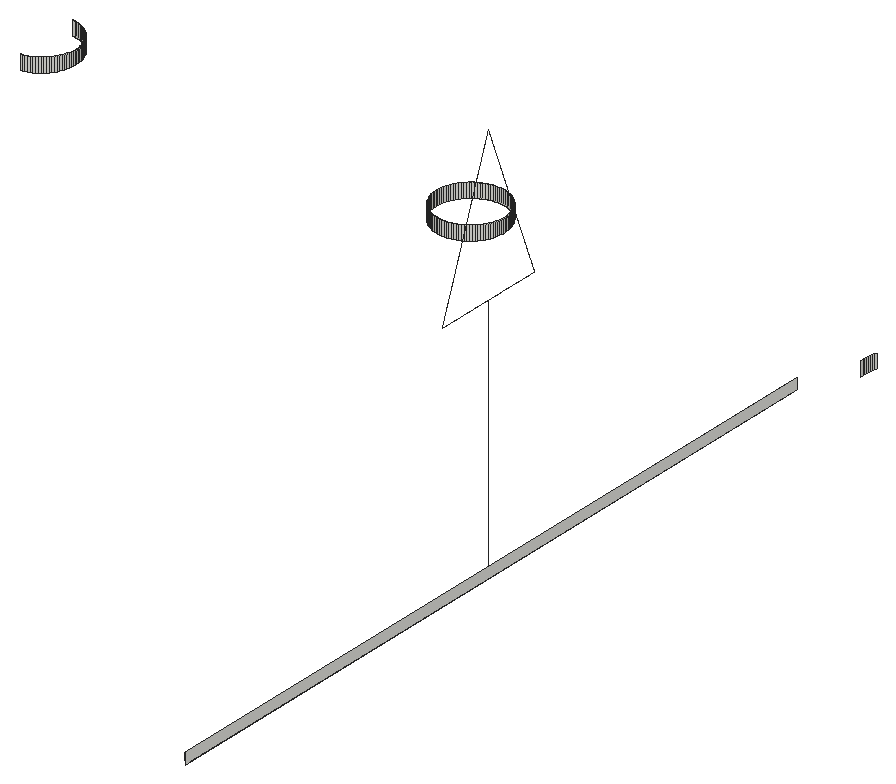
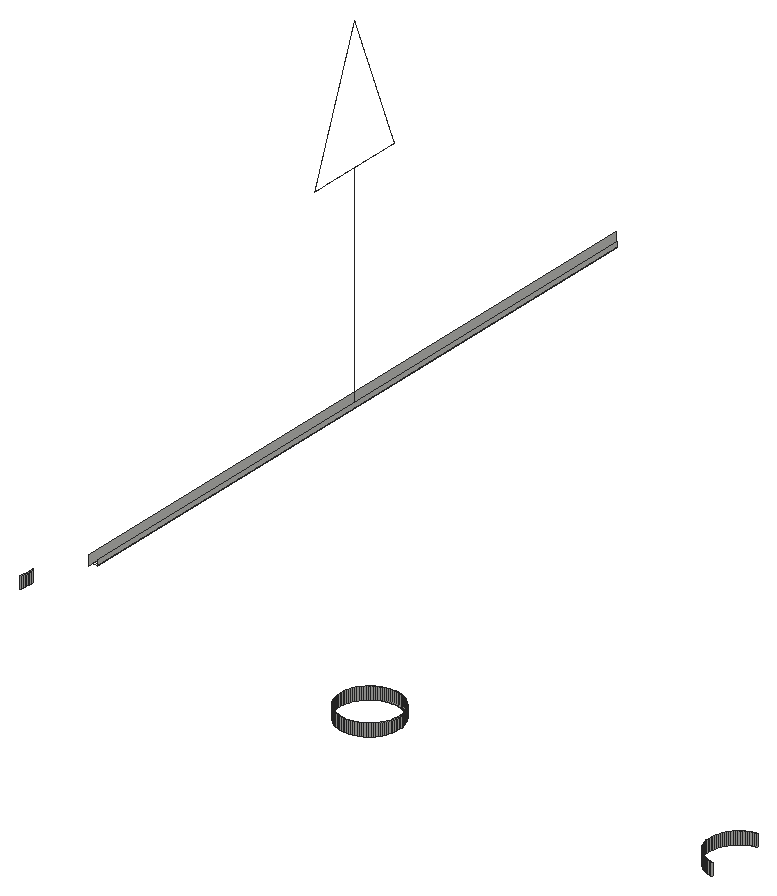
# SketchUp Ruby script. Lengths in inches.
U = 1.inch
M = Sketchup.active_model
def pt(a) = Geom::Point3d.new(a.map { |v| v * U })
def face(e, loops, mat)
  f = e.add_face(loops[0].map { |a| pt(a) })
  loops[1..].each { |l| e.add_face(l.map { |a| pt(a) }).erase! }
  f.material = f.back_material = mat if mat
  f
end
# faces: each face lists its corners as indices into pts; further lists are holes
def faces(e, pts, list, mat = nil) = list.each { |f| face(e, (f[0].is_a?(Array) ? f : [f]).map { |l| l.map { |i| pts[i] } }, mat) }
# xy, xz, yz: faces in a plane at the given z, y or x. An outline is a flat list of corners, or four numbers for a rectangle; further outlines are holes
def ring(l) = l.size == 4 ? [[l[0], l[1]], [l[2], l[1]], [l[2], l[3]], [l[0], l[3]]] : l.each_slice(2).to_a
def flat(e, list, mat, &to3) = list.each { |f| face(e, (f[0].is_a?(Array) ? f : [f]).map { |l| ring(l).map { |u, v| to3.(u, v) } }, mat) }
def xy(e, z, list, mat = nil) = flat(e, list, mat) { |x, y| [x, y, z] }
def xz(e, y, list, mat = nil) = flat(e, list, mat) { |x, z| [x, y, z] }
def yz(e, x, list, mat = nil) = flat(e, list, mat) { |y, z| [x, y, z] }
def lines(e, pts, list) = list.each { |a, b| e.add_line(pt(pts[a]), pt(pts[b])) }
# prism: a flat outline (further loops are holes) pulled along v
def prism(e, loops, v, mat = nil)
  f = face(e, loops, mat); d = Geom::Vector3d.new(v.map { |x| x * U })
  f.pushpull(f.normal.samedirection?(d) ? d.length : -d.length)
end
def box(e, o, s, mat = nil) = prism(e, [[o, [o[0] + s[0], o[1], o[2]], [o[0] + s[0], o[1] + s[1], o[2]], [o[0], o[1] + s[1], o[2]]]], [0, 0, s[2]], mat)
def at(x, y, z, deg = 0) = Geom::Transformation.translation(pt([x, y, z])) * Geom::Transformation.rotation(ORIGIN, Z_AXIS, deg.degrees)
def axes(o, x, y, z) = Geom::Transformation.new([*x, 0, *y, 0, *z, 0, *pt(o).to_a, 1])
def part(name) = M.definitions.add(name)
# library, detail: a bought-in or finely detailed component or shape, given as its bounding box
def library(name, o, s) = part(name).tap { |d| box(d.entities, o, s) }
def detail(e, o, s) = box(e.add_group.entities, o, s)
def put(e, d, t, mat = nil) = e.add_instance(d, t).tap { |i| i.material = mat if mat }
def group(e, t, mat = nil) = e.add_group.tap { |g| g.transformation = t; g.material = mat if mat }.entities
root = M.entities
c1 = part("Group84\#1")
p = [[0,0,0],[0,0,-43.36],[-21.49,0,-43.36],[139.88,-0.5,0],[-139.88,-0.5,0],[139.88,0.5,0],
  [139.88,0,0],[-139.88,0.5,0],[21.49,0,-43.36],[-139.88,0,0],[0,0,-70.19]]
lines(c1.entities,p,[[0,1],[1,2],[3,4],[5,6],[7,5],[1,8],[9,0],[0,6],[8,10],[4,9],[6,3],[2,10],
  [9,7]])
c2 = part("Rectangle Light")
put(c2.entities,c1,at(0,0,0))
xz(root,188,[[295.37,231.53,295.75,234]])
xz(root,200,[[295.37,231.53,295.75,234]])
yz(root,226.37,[[193.8125,231.53,194.1875,234]])
yz(root,289.5625,[[193.8125,231.53,194.1875,234]])
yz(root,301.56,[[193.8125,231.53,194.1875,234]])
yz(root,359.75,[[51,232,183,233]])
yz(root,360.75,[[50,232,184,234]])
yz(root,364.75,[[193.8125,231.53,194.1875,234]])
p = [[295,188.03,231.53],[294.62,188.07,231.53],[294.62,188.07,234],[295,188.03,234],[295.37,188,231.53],[295.37,188,234],
  [296.125,188.03,231.53],[295.75,188,231.53],[295.75,188,234],[296.125,188.03,234],[296.5,188.07,231.53],[296.5,188.07,234],
  [221.68,188.14,231.53],[221.31,188.07,231.53],[221.31,188.07,234],[221.68,188.14,234],[222.04,188.24,231.53],[222.04,188.24,234],
  [294.25,188.14,231.53],[293.89,188.24,231.53],[293.89,188.24,234],[294.25,188.14,234],[296.87,188.14,231.53],[296.87,188.14,234],
  [297.23,188.24,231.53],[297.23,188.24,234],[222.4,188.35,231.53],[222.4,188.35,234],[293.53,188.35,231.53],[293.53,188.35,234],
  [297.59,188.35,231.53],[297.59,188.35,234],[222.75,188.49,231.53],[222.75,188.49,234],[293.18,188.49,231.53],[293.18,188.49,234],
  [297.94,188.49,231.53],[297.94,188.49,234],[223.09,188.65,231.53],[223.09,188.65,234],[292.84,188.65,231.53],[292.84,188.65,234],
  [298.28,188.65,231.53],[298.28,188.65,234],[223.43,188.84,231.53],[223.43,188.84,234],[292.51,188.84,231.53],[292.51,188.84,234],
  [298.61,188.84,231.53],[298.61,188.84,234],[223.74,189.04,231.53],[223.74,189.04,234],[292.1875,189.04,231.53],[292.1875,189.04,234],
  [298.93,189.04,231.53],[298.93,189.04,234],[224.05,189.26,231.53],[224.05,189.26,234],[291.88,189.26,231.53],[291.88,189.26,234],
  [299.24,189.26,231.53],[299.24,189.26,234],[224.34,189.5,231.53],[224.34,189.5,234],[291.59,189.5,231.53],[291.59,189.5,234],
  [299.53,189.5,231.53],[299.53,189.5,234],[224.61,189.76,231.53],[224.61,189.76,234],[291.32,189.76,231.53],[291.32,189.76,234],
  [299.8,189.76,231.53],[299.8,189.76,234],[224.87,190.03,231.53],[224.87,190.03,234],[291.06,190.03,231.53],[291.06,190.03,234],
  [300.0625,190.03,231.53],[300.0625,190.03,234],[225.11,190.32,231.53],[225.11,190.32,234],[290.82,190.32,231.53],[290.82,190.32,234],
  [300.3,190.32,231.53],[300.3,190.32,234],[225.33,190.63,231.53],[225.33,190.63,234],[290.6,190.63,231.53],[290.6,190.63,234],
  [300.52,190.63,231.53],[300.52,190.63,234],[225.54,190.95,231.53],[225.54,190.95,234],[290.4,190.95,231.53],[290.4,190.95,234],
  [300.72,190.95,231.53],[300.72,190.95,234],[225.72,191.28,231.53],[225.72,191.28,234],[290.21,191.28,231.53],[290.21,191.28,234],
  [300.91,191.28,231.53],[300.91,191.28,234],[225.88,191.62,231.53],[225.88,191.62,234],[290.05,191.62,231.53],[290.05,191.62,234],
  [301.07,191.62,231.53],[301.07,191.62,234],[226.02,191.97,231.53],[226.02,191.97,234],[289.92,191.97,231.53],[289.92,191.97,234],
  [301.21,191.97,231.53],[301.21,191.97,234],[226.13,192.33,231.53],[226.13,192.33,234],[289.8,192.33,231.53],[289.8,192.33,234],
  [301.32,192.33,231.53],[301.32,192.33,234],[226.23,192.69,231.53],[226.23,192.69,234],[289.7,192.69,231.53],[289.7,192.69,234],
  [301.42,192.69,231.53],[301.42,192.69,234],[226.3,193.0625,231.53],[226.3,193.0625,234],[289.63,193.0625,231.53],[289.63,193.0625,234],
  [301.49,193.0625,231.53],[301.49,193.0625,234],[226.34,193.44,231.53],[226.34,193.44,234],[289.59,193.44,231.53],[289.59,193.44,234],
  [301.53,193.44,231.53],[301.53,193.44,234],[364.82,193.0625,231.53],[364.78,193.44,231.53],[364.78,193.44,234],[364.82,193.0625,234],
  [226.37,193.8125,231.53],[226.37,193.8125,234],[289.5625,193.8125,231.53],[289.5625,193.8125,234],[301.56,193.8125,231.53],[301.56,193.8125,234],
  [364.75,193.8125,231.53],[364.75,193.8125,234],[226.34,194.56,231.53],[226.37,194.1875,231.53],[226.37,194.1875,234],[226.34,194.56,234],
  [289.5625,194.1875,231.53],[289.59,194.56,231.53],[289.59,194.56,234],[289.5625,194.1875,234],[301.53,194.56,231.53],[301.56,194.1875,231.53],
  [301.56,194.1875,234],[301.53,194.56,234],[364.75,194.1875,231.53],[364.78,194.56,231.53],[364.78,194.56,234],[364.75,194.1875,234],
  [226.3,194.9375,231.53],[226.3,194.9375,234],[289.63,194.9375,231.53],[289.63,194.9375,234],[301.49,194.9375,231.53],[301.49,194.9375,234],
  [364.82,194.9375,231.53],[364.82,194.9375,234],[226.23,195.31,231.53],[226.23,195.31,234],[289.7,195.31,231.53],[289.7,195.31,234],
  [301.42,195.31,231.53],[301.42,195.31,234],[364.89,195.31,231.53],[364.89,195.31,234],[226.13,195.67,231.53],[226.13,195.67,234],
  [289.8,195.67,231.53],[289.8,195.67,234],[301.32,195.67,231.53],[301.32,195.67,234],[364.99,195.67,231.53],[364.99,195.67,234],
  [226.02,196.03,231.53],[226.02,196.03,234],[289.92,196.03,231.53],[289.92,196.03,234],[301.21,196.03,231.53],[301.21,196.03,234],
  [365.1,196.03,231.53],[365.1,196.03,234],[225.88,196.38,231.53],[225.88,196.38,234],[290.05,196.38,231.53],[290.05,196.38,234],
  [301.07,196.38,231.53],[301.07,196.38,234],[225.72,196.72,231.53],[225.72,196.72,234],[290.21,196.72,231.53],[290.21,196.72,234],
  [300.91,196.72,231.53],[300.91,196.72,234],[225.54,197.05,231.53],[225.54,197.05,234],[290.4,197.05,231.53],[290.4,197.05,234],
  [300.72,197.05,231.53],[300.72,197.05,234],[225.33,197.37,231.53],[225.33,197.37,234],[290.6,197.37,231.53],[290.6,197.37,234],
  [300.52,197.37,231.53],[300.52,197.37,234],[225.11,197.68,231.53],[225.11,197.68,234],[290.82,197.68,231.53],[290.82,197.68,234],
  [300.3,197.68,231.53],[300.3,197.68,234],[224.87,197.97,231.53],[224.87,197.97,234],[291.06,197.97,231.53],[291.06,197.97,234],
  [300.0625,197.97,231.53],[300.0625,197.97,234],[224.61,198.24,231.53],[224.61,198.24,234],[291.32,198.24,231.53],[291.32,198.24,234],
  [299.8,198.24,231.53],[299.8,198.24,234],[224.34,198.5,231.53],[224.34,198.5,234],[291.59,198.5,231.53],[291.59,198.5,234],
  [299.53,198.5,231.53],[299.53,198.5,234],[224.05,198.74,231.53],[224.05,198.74,234],[291.88,198.74,231.53],[291.88,198.74,234],
  [299.24,198.74,231.53],[299.24,198.74,234],[223.74,198.96,231.53],[223.74,198.96,234],[292.1875,198.96,231.53],[292.1875,198.96,234],
  [298.93,198.96,231.53],[298.93,198.96,234],[223.43,199.16,231.53],[223.43,199.16,234],[292.51,199.16,231.53],[292.51,199.16,234],
  [298.61,199.16,231.53],[298.61,199.16,234],[223.09,199.35,231.53],[223.09,199.35,234],[292.84,199.35,231.53],[292.84,199.35,234],
  [298.28,199.35,231.53],[298.28,199.35,234],[222.75,199.51,231.53],[222.75,199.51,234],[293.18,199.51,231.53],[293.18,199.51,234],
  [297.94,199.51,231.53],[297.94,199.51,234],[222.4,199.65,231.53],[222.4,199.65,234],[293.53,199.65,231.53],[293.53,199.65,234],
  [297.59,199.65,231.53],[297.59,199.65,234],[222.04,199.76,231.53],[222.04,199.76,234],[293.89,199.76,231.53],[293.89,199.76,234],
  [297.23,199.76,231.53],[297.23,199.76,234],[221.68,199.86,231.53],[221.68,199.86,234],[294.25,199.86,231.53],[294.25,199.86,234],
  [296.87,199.86,231.53],[296.87,199.86,234],[220.94,199.97,231.53],[221.31,199.93,231.53],[221.31,199.93,234],[220.94,199.97,234],
  [294.62,199.93,231.53],[294.62,199.93,234],[295,199.97,231.53],[295,199.97,234],[296.125,199.97,231.53],[296.5,199.93,231.53],
  [296.5,199.93,234],[296.125,199.97,234],[295.37,200,231.53],[295.37,200,234],[295.75,200,231.53],[295.75,200,234]]
faces(root,p,[[0,1,2,3],[4,0,3,5],[6,7,8,9],[10,6,9,11],[12,13,14,15],[16,12,15,17],[18,19,20,21],[1,18,21,2],
  [22,10,11,23],[24,22,23,25],[26,16,17,27],[19,28,29,20],[30,24,25,31],[32,26,27,33],[28,34,35,29],[36,30,31,37],
  [38,32,33,39],[34,40,41,35],[42,36,37,43],[44,38,39,45],[40,46,47,41],[48,42,43,49],[50,44,45,51],[46,52,53,47],
  [54,48,49,55],[56,50,51,57],[52,58,59,53],[60,54,55,61],[62,56,57,63],[58,64,65,59],[66,60,61,67],[68,62,63,69],
  [64,70,71,65],[72,66,67,73],[74,68,69,75],[70,76,77,71],[78,72,73,79],[80,74,75,81],[76,82,83,77],[84,78,79,85],
  [86,80,81,87],[82,88,89,83],[90,84,85,91],[92,86,87,93],[88,94,95,89],[96,90,91,97],[98,92,93,99],[94,100,101,95],
  [102,96,97,103],[104,98,99,105],[100,106,107,101],[108,102,103,109],[110,104,105,111],[106,112,113,107],[114,108,109,115],[116,110,111,117],
  [112,118,119,113],[120,114,115,121],[122,116,117,123],[118,124,125,119],[126,120,121,127],[128,122,123,129],[124,130,131,125],[132,126,127,133],
  [134,128,129,135],[130,136,137,131],[138,132,133,139],[140,141,142,143],[144,134,135,145],[136,146,147,137],[148,138,139,149],[141,150,151,142],
  [152,153,154,155],[156,157,158,159],[160,161,162,163],[164,165,166,167],[168,152,155,169],[157,170,171,158],[172,160,163,173],[165,174,175,166],
  [176,168,169,177],[170,178,179,171],[180,172,173,181],[174,182,183,175],[184,176,177,185],[178,186,187,179],[188,180,181,189],[182,190,191,183],
  [192,184,185,193],[186,194,195,187],[196,188,189,197],[190,198,199,191],[200,192,193,201],[194,202,203,195],[204,196,197,205],[206,200,201,207],
  [202,208,209,203],[210,204,205,211],[212,206,207,213],[208,214,215,209],[216,210,211,217],[218,212,213,219],[214,220,221,215],[222,216,217,223],
  [224,218,219,225],[220,226,227,221],[228,222,223,229],[230,224,225,231],[226,232,233,227],[234,228,229,235],[236,230,231,237],[232,238,239,233],
  [240,234,235,241],[242,236,237,243],[238,244,245,239],[246,240,241,247],[248,242,243,249],[244,250,251,245],[252,246,247,253],[254,248,249,255],
  [250,256,257,251],[258,252,253,259],[260,254,255,261],[256,262,263,257],[264,258,259,265],[266,260,261,267],[262,268,269,263],[270,264,265,271],
  [272,266,267,273],[268,274,275,269],[276,270,271,277],[278,272,273,279],[274,280,281,275],[282,276,277,283],[284,278,279,285],[280,286,287,281],
  [288,282,283,289],[290,284,285,291],[286,292,293,287],[294,288,289,295],[296,297,298,299],[297,290,291,298],[292,300,301,293],[300,302,303,301],
  [304,305,306,307],[305,294,295,306],[302,308,309,303],[310,304,307,311]])
put(root,c2,axes([360.25,117,232.01],[0,-0.47184,0],[-1,0,0],[0,0,-1]))
